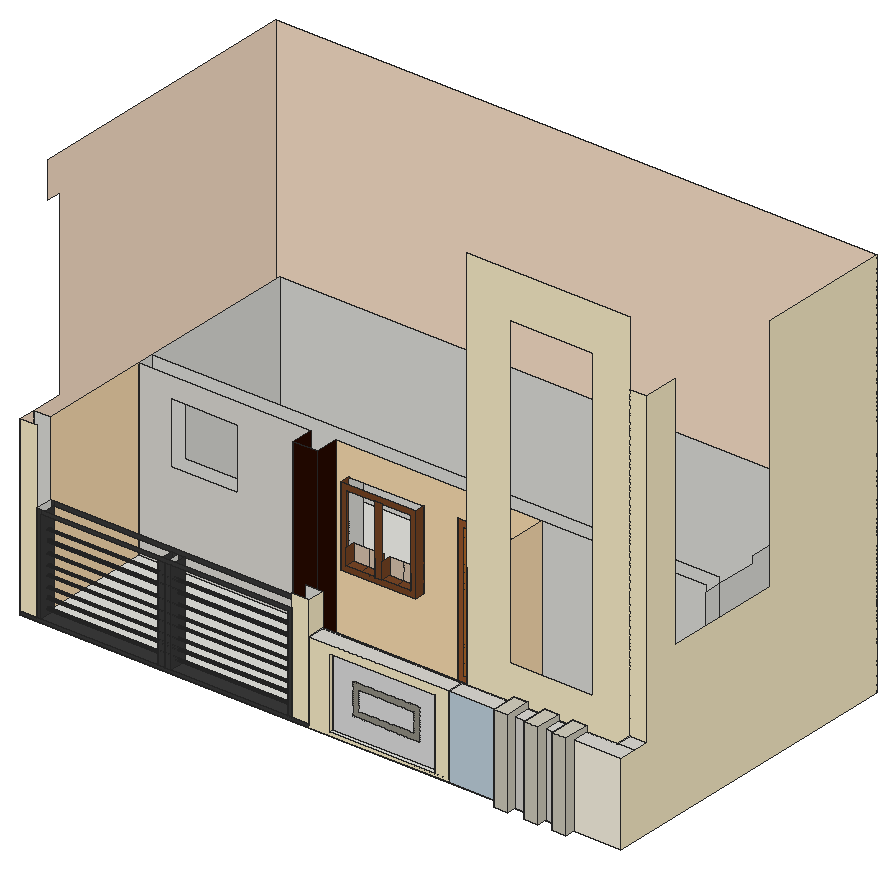
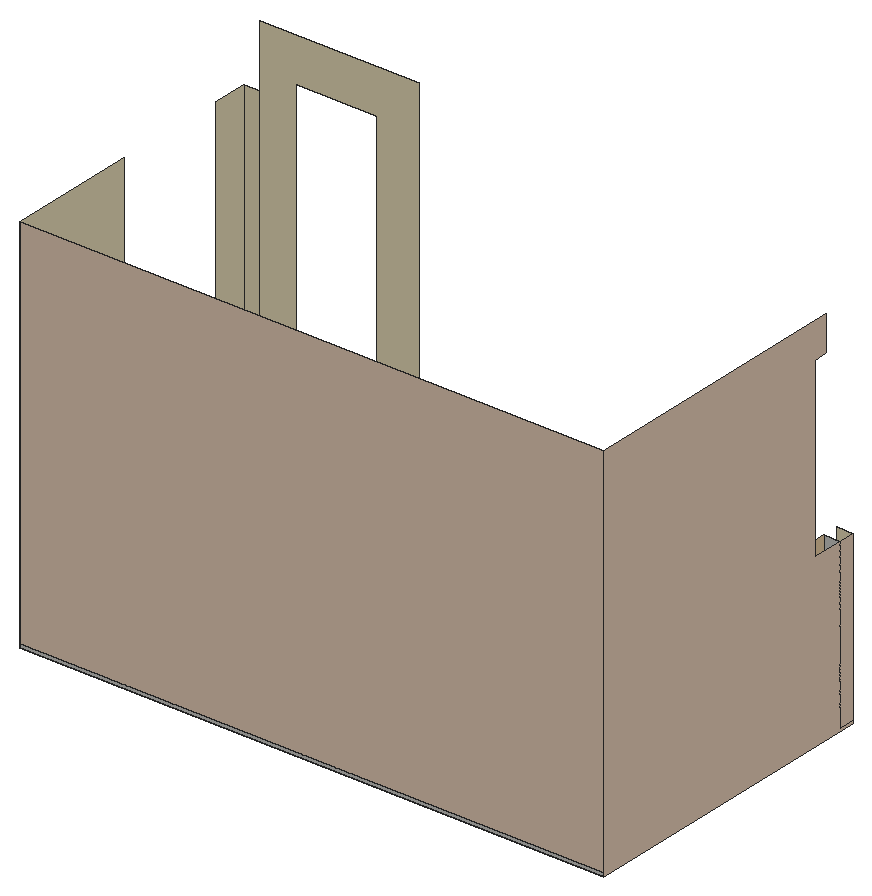
# SketchUp Ruby script. Lengths in inches.
U = 1.inch
M = Sketchup.active_model
def pt(a) = Geom::Point3d.new(a.map { |v| v * U })
def face(e, loops, mat)
  f = e.add_face(loops[0].map { |a| pt(a) })
  loops[1..].each { |l| e.add_face(l.map { |a| pt(a) }).erase! }
  f.material = f.back_material = mat if mat
  f
end
# faces: each face lists its corners as indices into pts; further lists are holes
def faces(e, pts, list, mat = nil) = list.each { |f| face(e, (f[0].is_a?(Array) ? f : [f]).map { |l| l.map { |i| pts[i] } }, mat) }
# xy, xz, yz: faces in a plane at the given z, y or x. An outline is a flat list of corners, or four numbers for a rectangle; further outlines are holes
def ring(l) = l.size == 4 ? [[l[0], l[1]], [l[2], l[1]], [l[2], l[3]], [l[0], l[3]]] : l.each_slice(2).to_a
def flat(e, list, mat, &to3) = list.each { |f| face(e, (f[0].is_a?(Array) ? f : [f]).map { |l| ring(l).map { |u, v| to3.(u, v) } }, mat) }
def xy(e, z, list, mat = nil) = flat(e, list, mat) { |x, y| [x, y, z] }
def xz(e, y, list, mat = nil) = flat(e, list, mat) { |x, z| [x, y, z] }
def yz(e, x, list, mat = nil) = flat(e, list, mat) { |y, z| [x, y, z] }
def lines(e, pts, list) = list.each { |a, b| e.add_line(pt(pts[a]), pt(pts[b])) }
# prism: a flat outline (further loops are holes) pulled along v
def prism(e, loops, v, mat = nil)
  f = face(e, loops, mat); d = Geom::Vector3d.new(v.map { |x| x * U })
  f.pushpull(f.normal.samedirection?(d) ? d.length : -d.length)
end
def box(e, o, s, mat = nil) = prism(e, [[o, [o[0] + s[0], o[1], o[2]], [o[0] + s[0], o[1] + s[1], o[2]], [o[0], o[1] + s[1], o[2]]]], [0, 0, s[2]], mat)
def at(x, y, z, deg = 0) = Geom::Transformation.translation(pt([x, y, z])) * Geom::Transformation.rotation(ORIGIN, Z_AXIS, deg.degrees)
def axes(o, x, y, z) = Geom::Transformation.new([*x, 0, *y, 0, *z, 0, *pt(o).to_a, 1])
def part(name) = M.definitions.add(name)
# library, detail: a bought-in or finely detailed component or shape, given as its bounding box
def library(name, o, s) = part(name).tap { |d| box(d.entities, o, s) }
def detail(e, o, s) = box(e.add_group.entities, o, s)
def put(e, d, t, mat = nil) = e.add_instance(d, t).tap { |i| i.material = mat if mat }
def group(e, t, mat = nil) = e.add_group.tap { |g| g.transformation = t; g.material = mat if mat }.entities
root = M.entities
M.materials.add("[Color B08]").color = [40, 10, 0]
M.materials.add("[Color C01]").color = [221, 199, 177]
M.materials.add("[Color C01]1").color = [255, 229, 204]
M.materials.add("[Color D01]").color = [255, 242, 204]
M.materials.add("[Color M01]").color = [226, 226, 226]
M.materials.add("[Color M07]").color = [58, 58, 58]
M.materials.add("[Formica Beige]").color = [255, 225, 180]
M.materials.add("[Formica Graystone]").color = [211, 207, 191]
M.materials.add("[Formica Graystone]1").color = [255, 249, 231]
M.materials.add("[Formica Graystone]2").color = [149, 146, 135]
M.materials.add("[Formica Laminate Dark]").color = [50, 53, 60]
M.materials.add("[Marble Carrara Gold Floor Tile]").color = [225, 223, 217]
M.materials.add("[Terrazzo Light Blue]").color = [196, 214, 227]
M.materials.add("[Terrazzo Tile Light]").color = [219, 217, 210]
M.materials.add("[Wood Bamboo]").color = [177, 105, 43]
M.materials.add("[Wood Cherry Original]").color = [152, 86, 42]
M.materials.add("[Wood Floor Light]").color = [204, 176, 127]
M.materials.add("[Wood Veneer 01]").color = [120, 70, 37]
xy(root,0,[[1538.08,0,1538.08,25.9375,0,25.9375,0,938.08,1713.03,938.08,1713.03,25.9375,1578.55,25.9375,1578.55,0],[1370.58,0,1411.05,25.9375],[1458.08,0,1498.55,25.9375]])
xy(root,9,[[0,25.9375,0,73.63,1665.33,73.63,1665.33,119.17,1198.27,119.17,1198.27,388.54,609.42,388.54,609.42,324.79,539.84,324.79,539.84,388.54,47.7,388.54,47.7,25.9375],[47.7,25.9375,58.17,73.63],[392.86,25.9375,411.53,73.63],[411.53,25.9375,430.19,73.63],[763.2,25.9375,775.53,73.63],
  [775.53,25.9375,824.4,73.63],[882.08,25.9375,1183.86,38.5625],[1183.86,25.9375,1222.55,73.63],[882.08,38.5625,1183.86,73.63],[958.75,388.54,1164.68,436.38],
  [47.7,436.38,1665.33,890.39]])
xy(root,9,[[58.17,25.9375,392.86,73.63],[430.19,25.9375,763.2,73.63]],"[Color M07]")
xy(root,195.52,[[648.52,388.54,860.65,436.38]])
xy(root,195.52,[[648.52,359.29,860.65,388.54]],"[Wood Veneer 01]")
xy(root,209.32,[[882.08,25.9375,1183.86,38.5625]],"[Color D01]")
xy(root,209.8125,[[662.82,359.29,704.31,388.54],[704.31,359.29,745.81,388.54],[764.54,359.29,805.45,388.54],[805.45,359.29,846.36,388.54]],"[Wood Veneer 01]")
xy(root,233.1875,[[1370.58,25.9375,1411.05,73.63],[1458.08,25.9375,1498.55,73.63]])
xy(root,233.1875,[[824.4,25.9375,1222.55,73.63],[1222.55,25.9375,1370.58,73.63],[1411.05,25.9375,1458.08,73.63],[1498.55,25.9375,1538.08,73.63],[1578.55,25.9375,1713.03,73.63],
  [1665.33,73.63,1713.03,119.17]],"[Terrazzo Tile Light]")
xy(root,249.75,[[1370.58,0,1411.05,73.63],[1458.08,0,1498.55,73.63],[1538.08,0,1578.55,73.63]],"[Formica Graystone]")
xz(root,0,[[1370.58,0,1411.05,249.75],[1458.08,0,1498.55,249.75],[1538.08,0,1578.55,249.75]],"[Formica Graystone]")
xz(root,25.9375,[[1370.58,0,1411.05,233.1875],[1458.08,0,1498.55,233.1875]])
xz(root,25.9375,[[824.4,0,1222.55,0,1222.55,9,882.08,9,882.08,209.32,1183.86,209.32,1183.86,9,1222.55,9,1222.55,233.1875,824.4,233.1875],[0,9,47.7,500.125],[775.53,9,824.4,326.25]],"[Color D01]")
xz(root,25.9375,[[0,0,824.4,9],[47.7,9,58.17,288.4375],[763.2,9,775.53,9,775.53,288.4375,58.17,288.4375,58.17,276.5625,763.2,276.5625],[392.86,9,411.53,276.5625],[411.53,9,430.19,276.5625]],"[Color M07]")
xz(root,25.9375,[[1578.55,0,1713.03,233.1875]],"[Formica Graystone]1")
xz(root,25.9375,[[1222.55,0,1370.58,233.1875]],"[Terrazzo Light Blue]")
xz(root,25.9375,[[1411.05,0,1458.08,233.1875],[1498.55,0,1538.08,233.1875]],"[Terrazzo Tile Light]")
xz(root,38.5625,[[[882.08,9,1183.86,209.32],[939.22,64.12,1130.16,154.99]],[957.24,82.13,1112.14,136.97]],"[Color M01]")
xz(root,38.5625,[[[939.22,64.12,1130.16,154.99],[957.24,82.13,1112.14,136.97]]],"[Formica Graystone]2")
xz(root,73.63,[[0,9,47.7,500.125],[775.53,9,824.4,326.25],[824.4,9,882.08,233.1875],[1183.86,9,1183.86,209.32,882.08,209.32,882.08,233.1875,1222.55,233.1875,1222.55,9],[882.08,9,1183.86,209.32]])
xz(root,73.63,[[47.7,9,58.17,288.4375],[763.2,9,763.2,276.5625,58.17,276.5625,58.17,288.4375,775.53,288.4375,775.53,9],[392.86,9,411.53,276.5625],[411.53,9,430.19,276.5625]],"[Color M07]")
xz(root,73.63,[[1222.55,9,1222.55,233.1875,1538.08,233.1875,1538.08,249.75,1578.55,249.75,1578.55,233.1875,1665.33,233.1875,1665.33,9],[1370.58,233.1875,1411.05,249.75],[1458.08,233.1875,1498.55,249.75]],"[Formica Graystone]")
xz(root,119.17,[[[1198.27,9,1665.33,1305.375],[1322.15,298.625,1559.21,1175.6875]],[1665.33,233.1875,1713.03,1119.0625]],"[Color D01]")
xz(root,324.79,[[539.84,9,609.42,500.125]],"[Color B08]")
xz(root,359.29,[[[648.52,195.52,860.65,420.08],[662.82,209.8125,846.36,405.79]],[745.81,209.8125,764.54,405.79]],"[Wood Veneer 01]")
xz(root,388.54,[[1198.27,9,1665.33,500.125]])
xz(root,388.54,[[662.82,209.8125,704.31,256.87],[704.31,209.8125,745.81,256.87],[764.54,209.8125,805.45,256.87],[805.45,209.8125,846.36,256.87]],"[Color C01]")
xz(root,388.54,[[[609.42,9,958.75,9,958.75,423.9375,1164.68,423.9375,1164.68,9,1198.27,9,1198.27,500.125,609.42,500.125],[648.52,195.52,860.65,420.08]]],"[Formica Beige]")
xz(root,388.54,[[[47.7,9,539.84,500.125],[139.94,267,331.76,443.06]]],"[Marble Carrara Gold Floor Tile]")
xz(root,388.54,[[[976.52,26.77,1146.91,406.17],[984.3,166.91,996.99,249.85]]],"[Wood Bamboo]")
xz(root,388.54,[[[958.75,9,1164.68,423.9375],[976.52,26.77,1146.91,406.17]]],"[Wood Cherry Original]")
xz(root,388.54,[[984.3,166.91,996.99,249.85]],"[Wood Floor Light]")
xz(root,436.38,[[[47.7,9,47.7,500.125,1665.33,500.125,1665.33,9,1164.68,9,1164.68,423.9375,958.75,423.9375,958.75,9],[648.52,195.52,860.65,420.08],[139.94,267,331.76,443.06]]])
xz(root,890.39,[[47.7,9,1665.33,500.125]])
xz(root,938.08,[[0,0,1713.03,9]])
xz(root,938.08,[[0,9,1713.03,1119.0625]],"[Color C01]1")
yz(root,0,[[25.9375,0,25.9375,9,73.63,9,73.63,500.125,166.1,500.125,166.1,1016.9375,122.54,1016.9375,122.54,1119.0625,938.08,1119.0625,938.08,0],[25.9375,9,73.63,500.125]],"[Color C01]1")
yz(root,47.7,[[25.9375,9,73.63,288.4375],[388.54,9,436.38,500.125],[436.38,9,890.39,500.125]])
yz(root,47.7,[[73.63,9,388.54,500.125]],"[Formica Beige]")
yz(root,58.17,[[51.27,21.94,50.49,22.04,49.77,22.34,49.15,22.82,48.67,23.44,48.37,24.16,48.27,24.94,48.37,25.72,48.67,26.44,49.15,27.0625,49.77,27.54,50.49,27.84,51.27,27.94,52.04,27.84,52.77,27.54,53.39,27.0625,53.87,26.44,54.17,25.72,54.27,24.94,54.17,24.16,53.87,23.44,53.39,22.82,52.77,22.34,52.04,22.04],[51.27,49.25,50.49,49.35,49.77,49.65,49.15,50.13,48.67,50.75,48.37,51.48,48.27,52.25,48.37,53.03,48.67,53.75,49.15,54.375,49.77,54.85,50.49,55.15,51.27,55.25,52.04,55.15,52.77,54.85,53.39,54.375,53.87,53.75,54.17,53.03,54.27,52.25,54.17,51.48,53.87,50.75,53.39,50.13,52.77,49.65,52.04,49.35],[51.27,76.69,50.49,76.79,49.77,77.09,49.15,77.57,48.67,78.19,48.37,78.91,48.27,79.69,48.37,80.47,48.67,81.19,49.15,81.8125,49.77,82.29,50.49,82.59,51.27,82.69,52.04,82.59,52.77,82.29,53.39,81.8125,53.87,81.19,54.17,80.47,54.27,79.69,54.17,78.91,53.87,78.19,53.39,77.57,52.77,77.09,52.04,76.79],[51.27,107.44,50.49,107.54,49.77,107.84,49.15,108.32,48.67,108.94,48.37,109.66,48.27,110.44,48.37,111.22,48.67,111.94,49.15,112.5625,49.77,113.04,50.49,113.34,51.27,113.44,52.04,113.34,52.77,113.04,53.39,112.5625,53.87,111.94,54.17,111.22,54.27,110.44,54.17,109.66,53.87,108.94,53.39,108.32,52.77,107.84,52.04,107.54],[51.27,132.75,50.49,132.85,49.77,133.15,49.15,133.63,48.67,134.25,48.37,134.98,48.27,135.75,48.37,136.53,48.67,137.25,49.15,137.875,49.77,138.35,50.49,138.65,51.27,138.75,52.04,138.65,52.77,138.35,53.39,137.875,53.87,137.25,54.17,136.53,54.27,135.75,54.17,134.98,53.87,134.25,53.39,133.63,52.77,133.15,52.04,132.85],
  [51.27,163.5,50.49,163.6,49.77,163.9,49.15,164.38,48.67,165,48.37,165.73,48.27,166.5,48.37,167.28,48.67,168,49.15,168.625,49.77,169.1,50.49,169.4,51.27,169.5,52.04,169.4,52.77,169.1,53.39,168.625,53.87,168,54.17,167.28,54.27,166.5,54.17,165.73,53.87,165,53.39,164.38,52.77,163.9,52.04,163.6],[51.27,195.56,50.49,195.67,49.77,195.97,49.15,196.44,48.67,197.06,48.37,197.79,48.27,198.56,48.37,199.34,48.67,200.06,49.15,200.6875,49.77,201.16,50.49,201.46,51.27,201.56,52.04,201.46,52.77,201.16,53.39,200.6875,53.87,200.06,54.17,199.34,54.27,198.56,54.17,197.79,53.87,197.06,53.39,196.44,52.77,195.97,52.04,195.67],[51.27,225.44,50.49,225.54,49.77,225.84,49.15,226.32,48.67,226.94,48.37,227.66,48.27,228.44,48.37,229.22,48.67,229.94,49.15,230.5625,49.77,231.04,50.49,231.34,51.27,231.44,52.04,231.34,52.77,231.04,53.39,230.5625,53.87,229.94,54.17,229.22,54.27,228.44,54.17,227.66,53.87,226.94,53.39,226.32,52.77,225.84,52.04,225.54]])
yz(root,58.17,[[[25.9375,9,73.63,276.5625],[51.27,21.94,50.49,22.04,49.77,22.34,49.15,22.82,48.67,23.44,48.37,24.16,48.27,24.94,48.37,25.72,48.67,26.44,49.15,27.0625,49.77,27.54,50.49,27.84,51.27,27.94,52.04,27.84,52.77,27.54,53.39,27.0625,53.87,26.44,54.17,25.72,54.27,24.94,54.17,24.16,53.87,23.44,53.39,22.82,52.77,22.34,52.04,22.04],[51.27,225.44,50.49,225.54,49.77,225.84,49.15,226.32,48.67,226.94,48.37,227.66,48.27,228.44,48.37,229.22,48.67,229.94,49.15,230.5625,49.77,231.04,50.49,231.34,51.27,231.44,52.04,231.34,52.77,231.04,53.39,230.5625,53.87,229.94,54.17,229.22,54.27,228.44,54.17,227.66,53.87,226.94,53.39,226.32,52.77,225.84,52.04,225.54],[51.27,49.25,50.49,49.35,49.77,49.65,49.15,50.13,48.67,50.75,48.37,51.48,48.27,52.25,48.37,53.03,48.67,53.75,49.15,54.375,49.77,54.85,50.49,55.15,51.27,55.25,52.04,55.15,52.77,54.85,53.39,54.375,53.87,53.75,54.17,53.03,54.27,52.25,54.17,51.48,53.87,50.75,53.39,50.13,52.77,49.65,52.04,49.35],[51.27,195.56,50.49,195.67,49.77,195.97,49.15,196.44,48.67,197.06,48.37,197.79,48.27,198.56,48.37,199.34,48.67,200.06,49.15,200.6875,49.77,201.16,50.49,201.46,51.27,201.56,52.04,201.46,52.77,201.16,53.39,200.6875,53.87,200.06,54.17,199.34,54.27,198.56,54.17,197.79,53.87,197.06,53.39,196.44,52.77,195.97,52.04,195.67],[51.27,107.44,50.49,107.54,49.77,107.84,49.15,108.32,48.67,108.94,48.37,109.66,48.27,110.44,48.37,111.22,48.67,111.94,49.15,112.5625,49.77,113.04,50.49,113.34,51.27,113.44,52.04,113.34,52.77,113.04,53.39,112.5625,53.87,111.94,54.17,111.22,54.27,110.44,54.17,109.66,53.87,108.94,53.39,108.32,52.77,107.84,52.04,107.54],[51.27,163.5,50.49,163.6,49.77,163.9,49.15,164.38,48.67,165,48.37,165.73,48.27,166.5,48.37,167.28,48.67,168,49.15,168.625,49.77,169.1,50.49,169.4,51.27,169.5,52.04,169.4,52.77,169.1,53.39,168.625,53.87,168,54.17,167.28,54.27,166.5,54.17,165.73,53.87,165,53.39,164.38,52.77,163.9,52.04,163.6],[51.27,132.75,50.49,132.85,49.77,133.15,49.15,133.63,48.67,134.25,48.37,134.98,48.27,135.75,48.37,136.53,48.67,137.25,49.15,137.875,49.77,138.35,50.49,138.65,51.27,138.75,52.04,138.65,52.77,138.35,53.39,137.875,53.87,137.25,54.17,136.53,54.27,135.75,54.17,134.98,53.87,134.25,53.39,133.63,52.77,133.15,52.04,132.85],[51.27,76.69,50.49,76.79,49.77,77.09,49.15,77.57,48.67,78.19,48.37,78.91,48.27,79.69,48.37,80.47,48.67,81.19,49.15,81.8125,49.77,82.29,50.49,82.59,51.27,82.69,52.04,82.59,52.77,82.29,53.39,81.8125,53.87,81.19,54.17,80.47,54.27,79.69,54.17,78.91,53.87,78.19,53.39,77.57,52.77,77.09,52.04,76.79],[51.27,251.25,50.49,251.35,49.77,251.65,49.15,252.13,48.67,252.75,48.37,253.48,48.27,254.25,48.37,255.03,48.67,255.75,49.15,256.375,49.77,256.85,50.49,257.15,51.27,257.25,52.04,257.15,52.77,256.85,53.39,256.375,53.87,255.75,54.17,255.03,54.27,254.25,54.17,253.48,53.87,252.75,53.39,252.13,52.77,251.65,52.04,251.35]]],"[Color M07]")
yz(root,392.86,[[25.9375,9,73.63,276.5625]],"[Color M07]")
yz(root,411.53,[[25.9375,9,73.63,276.5625]])
yz(root,430.19,[[25.9375,9,73.63,276.5625]],"[Color M07]")
yz(root,539.84,[[324.79,9,388.54,500.125]],"[Color B08]")
yz(root,609.42,[[324.79,9,388.54,500.125]],"[Color B08]")
yz(root,648.52,[[388.54,195.52,436.38,420.08]])
yz(root,648.52,[[359.29,195.52,388.54,420.08]],"[Wood Veneer 01]")
yz(root,662.82,[[359.29,209.8125,388.54,256.87]],"[Wood Veneer 01]")
yz(root,745.81,[[359.29,209.8125,388.54,256.87]],"[Wood Veneer 01]")
yz(root,763.2,[[[25.9375,9,73.63,276.5625],[51.27,251.25,52.04,251.35,52.77,251.65,53.39,252.13,53.87,252.75,54.17,253.48,54.27,254.25,54.17,255.03,53.87,255.75,53.39,256.375,52.77,256.85,52.04,257.15,51.27,257.25,50.49,257.15,49.77,256.85,49.15,256.375,48.67,255.75,48.37,255.03,48.27,254.25,48.37,253.48,48.67,252.75,49.15,252.13,49.77,251.65,50.49,251.35],[51.27,225.44,52.04,225.54,52.77,225.84,53.39,226.32,53.87,226.94,54.17,227.66,54.27,228.44,54.17,229.22,53.87,229.94,53.39,230.5625,52.77,231.04,52.04,231.34,51.27,231.44,50.49,231.34,49.77,231.04,49.15,230.5625,48.67,229.94,48.37,229.22,48.27,228.44,48.37,227.66,48.67,226.94,49.15,226.32,49.77,225.84,50.49,225.54],[51.27,195.56,52.04,195.67,52.77,195.97,53.39,196.44,53.87,197.06,54.17,197.79,54.27,198.56,54.17,199.34,53.87,200.06,53.39,200.6875,52.77,201.16,52.04,201.46,51.27,201.56,50.49,201.46,49.77,201.16,49.15,200.6875,48.67,200.06,48.37,199.34,48.27,198.56,48.37,197.79,48.67,197.06,49.15,196.44,49.77,195.97,50.49,195.67],[51.27,163.5,52.04,163.6,52.77,163.9,53.39,164.38,53.87,165,54.17,165.73,54.27,166.5,54.17,167.28,53.87,168,53.39,168.625,52.77,169.1,52.04,169.4,51.27,169.5,50.49,169.4,49.77,169.1,49.15,168.625,48.67,168,48.37,167.28,48.27,166.5,48.37,165.73,48.67,165,49.15,164.38,49.77,163.9,50.49,163.6],[51.27,132.75,52.04,132.85,52.77,133.15,53.39,133.63,53.87,134.25,54.17,134.98,54.27,135.75,54.17,136.53,53.87,137.25,53.39,137.875,52.77,138.35,52.04,138.65,51.27,138.75,50.49,138.65,49.77,138.35,49.15,137.875,48.67,137.25,48.37,136.53,48.27,135.75,48.37,134.98,48.67,134.25,49.15,133.63,49.77,133.15,50.49,132.85],[51.27,107.44,52.04,107.54,52.77,107.84,53.39,108.32,53.87,108.94,54.17,109.66,54.27,110.44,54.17,111.22,53.87,111.94,53.39,112.5625,52.77,113.04,52.04,113.34,51.27,113.44,50.49,113.34,49.77,113.04,49.15,112.5625,48.67,111.94,48.37,111.22,48.27,110.44,48.37,109.66,48.67,108.94,49.15,108.32,49.77,107.84,50.49,107.54],[51.27,76.69,52.04,76.79,52.77,77.09,53.39,77.57,53.87,78.19,54.17,78.91,54.27,79.69,54.17,80.47,53.87,81.19,53.39,81.8125,52.77,82.29,52.04,82.59,51.27,82.69,50.49,82.59,49.77,82.29,49.15,81.8125,48.67,81.19,48.37,80.47,48.27,79.69,48.37,78.91,48.67,78.19,49.15,77.57,49.77,77.09,50.49,76.79],[51.27,49.25,52.04,49.35,52.77,49.65,53.39,50.13,53.87,50.75,54.17,51.48,54.27,52.25,54.17,53.03,53.87,53.75,53.39,54.375,52.77,54.85,52.04,55.15,51.27,55.25,50.49,55.15,49.77,54.85,49.15,54.375,48.67,53.75,48.37,53.03,48.27,52.25,48.37,51.48,48.67,50.75,49.15,50.13,49.77,49.65,50.49,49.35],[51.27,21.94,52.04,22.04,52.77,22.34,53.39,22.82,53.87,23.44,54.17,24.16,54.27,24.94,54.17,25.72,53.87,26.44,53.39,27.0625,52.77,27.54,52.04,27.84,51.27,27.94,50.49,27.84,49.77,27.54,49.15,27.0625,48.67,26.44,48.37,25.72,48.27,24.94,48.37,24.16,48.67,23.44,49.15,22.82,49.77,22.34,50.49,22.04]]],"[Color M07]")
yz(root,764.54,[[359.29,209.8125,388.54,256.87]],"[Wood Veneer 01]")
yz(root,775.53,[[25.9375,9,73.63,288.4375]])
yz(root,824.4,[[25.9375,9,73.63,233.1875]])
yz(root,824.4,[[25.9375,233.1875,73.63,326.25]],"[Color D01]")
yz(root,846.36,[[359.29,209.8125,388.54,256.87]],"[Wood Veneer 01]")
yz(root,860.65,[[388.54,195.52,436.38,420.08]])
yz(root,860.65,[[359.29,195.52,388.54,420.08]],"[Wood Veneer 01]")
yz(root,882.08,[[38.5625,9,73.63,209.32]])
yz(root,882.08,[[25.9375,9,38.5625,209.32]],"[Color D01]")
yz(root,958.75,[[388.54,9,436.38,423.9375]])
yz(root,1164.68,[[388.54,9,436.38,423.9375]])
yz(root,1183.86,[[38.5625,9,73.63,209.32]])
yz(root,1183.86,[[25.9375,9,38.5625,209.32]],"[Color D01]")
yz(root,1198.27,[[119.17,9,388.54,500.125]],"[Formica Beige]")
yz(root,1222.55,[[25.9375,9,73.63,233.1875]])
yz(root,1370.58,[[0,0,0,249.75,73.63,249.75,73.63,233.1875,25.9375,233.1875,25.9375,0]],"[Formica Graystone]")
yz(root,1411.05,[[0,0,25.9375,0,25.9375,233.1875,73.63,233.1875,73.63,249.75,0,249.75]],"[Formica Graystone]")
yz(root,1458.08,[[0,0,0,249.75,73.63,249.75,73.63,233.1875,25.9375,233.1875,25.9375,0]],"[Formica Graystone]")
yz(root,1498.55,[[0,0,25.9375,0,25.9375,233.1875,73.63,233.1875,73.63,249.75,0,249.75]],"[Formica Graystone]")
yz(root,1538.08,[[0,0,0,249.75,73.63,249.75,73.63,233.1875,25.9375,233.1875,25.9375,0]],"[Formica Graystone]")
yz(root,1578.55,[[0,0,25.9375,0,25.9375,233.1875,73.63,233.1875,73.63,249.75,0,249.75]],"[Formica Graystone]")
yz(root,1665.33,[[73.63,9,119.17,233.1875],[388.54,9,436.38,481.82],[436.38,9,436.38,481.82,557.62,481.82,557.62,500.125,890.39,500.125,890.39,9]])
yz(root,1713.03,[[25.9375,0,938.08,0,938.08,1119.0625,557.62,1119.0625,557.62,438.77,219.81,438.77,219.81,1119.0625,119.17,1119.0625,119.17,233.1875,25.9375,233.1875]],"[Color D01]")
p = [[58.17,50.49,22.04],[58.17,51.27,21.94],[763.2,51.27,21.94],[763.2,50.49,22.04],[58.17,52.04,22.04],[763.2,52.04,22.04],
  [58.17,49.77,22.34],[763.2,49.77,22.34],[58.17,52.77,22.34],[763.2,52.77,22.34],[58.17,49.15,22.82],[763.2,49.15,22.82],
  [58.17,53.39,22.82],[763.2,53.39,22.82],[58.17,48.67,23.44],[763.2,48.67,23.44],[58.17,53.87,23.44],[763.2,53.87,23.44],
  [58.17,48.37,24.16],[763.2,48.37,24.16],[58.17,54.17,24.16],[763.2,54.17,24.16],[58.17,48.27,24.94],[763.2,48.27,24.94],
  [58.17,54.27,24.94],[763.2,54.27,24.94],[58.17,48.37,25.72],[763.2,48.37,25.72],[58.17,54.17,25.72],[763.2,54.17,25.72],
  [58.17,48.67,26.44],[763.2,48.67,26.44],[58.17,53.87,26.44],[763.2,53.87,26.44],[58.17,49.15,27.0625],[763.2,49.15,27.0625],
  [58.17,53.39,27.0625],[763.2,53.39,27.0625],[58.17,49.77,27.54],[763.2,49.77,27.54],[58.17,52.77,27.54],[763.2,52.77,27.54],
  [58.17,50.49,27.84],[763.2,50.49,27.84],[58.17,52.04,27.84],[763.2,52.04,27.84],[58.17,51.27,27.94],[763.2,51.27,27.94],
  [58.17,50.49,49.35],[58.17,51.27,49.25],[763.2,51.27,49.25],[763.2,50.49,49.35],[58.17,52.04,49.35],[763.2,52.04,49.35],
  [58.17,49.77,49.65],[763.2,49.77,49.65],[58.17,52.77,49.65],[763.2,52.77,49.65],[58.17,49.15,50.13],[763.2,49.15,50.13],
  [58.17,53.39,50.13],[763.2,53.39,50.13],[58.17,48.67,50.75],[763.2,48.67,50.75],[58.17,53.87,50.75],[763.2,53.87,50.75],
  [58.17,48.37,51.48],[763.2,48.37,51.48],[58.17,54.17,51.48],[763.2,54.17,51.48],[58.17,48.27,52.25],[763.2,48.27,52.25],
  [58.17,54.27,52.25],[763.2,54.27,52.25],[58.17,48.37,53.03],[763.2,48.37,53.03],[58.17,54.17,53.03],[763.2,54.17,53.03],
  [58.17,48.67,53.75],[763.2,48.67,53.75],[58.17,53.87,53.75],[763.2,53.87,53.75],[58.17,49.15,54.375],[763.2,49.15,54.375],
  [58.17,53.39,54.375],[763.2,53.39,54.375],[58.17,49.77,54.85],[763.2,49.77,54.85],[58.17,52.77,54.85],[763.2,52.77,54.85],
  [58.17,50.49,55.15],[763.2,50.49,55.15],[58.17,52.04,55.15],[763.2,52.04,55.15],[58.17,51.27,55.25],[763.2,51.27,55.25],
  [58.17,50.49,76.79],[58.17,51.27,76.69],[763.2,51.27,76.69],[763.2,50.49,76.79],[58.17,52.04,76.79],[763.2,52.04,76.79],
  [58.17,49.77,77.09],[763.2,49.77,77.09],[58.17,52.77,77.09],[763.2,52.77,77.09],[58.17,49.15,77.57],[763.2,49.15,77.57],
  [58.17,53.39,77.57],[763.2,53.39,77.57],[58.17,48.67,78.19],[763.2,48.67,78.19],[58.17,53.87,78.19],[763.2,53.87,78.19],
  [58.17,48.37,78.91],[763.2,48.37,78.91],[58.17,54.17,78.91],[763.2,54.17,78.91],[58.17,48.27,79.69],[763.2,48.27,79.69],
  [58.17,54.27,79.69],[763.2,54.27,79.69],[58.17,48.37,80.47],[763.2,48.37,80.47],[58.17,54.17,80.47],[763.2,54.17,80.47],
  [58.17,48.67,81.19],[763.2,48.67,81.19],[58.17,53.87,81.19],[763.2,53.87,81.19],[58.17,49.15,81.8125],[763.2,49.15,81.8125],
  [58.17,53.39,81.8125],[763.2,53.39,81.8125],[58.17,49.77,82.29],[763.2,49.77,82.29],[58.17,52.77,82.29],[763.2,52.77,82.29],
  [58.17,50.49,82.59],[763.2,50.49,82.59],[58.17,52.04,82.59],[763.2,52.04,82.59],[58.17,51.27,82.69],[763.2,51.27,82.69],
  [58.17,50.49,107.54],[58.17,51.27,107.44],[763.2,51.27,107.44],[763.2,50.49,107.54],[58.17,52.04,107.54],[763.2,52.04,107.54],
  [58.17,49.77,107.84],[763.2,49.77,107.84],[58.17,52.77,107.84],[763.2,52.77,107.84],[58.17,49.15,108.32],[763.2,49.15,108.32],
  [58.17,53.39,108.32],[763.2,53.39,108.32],[58.17,48.67,108.94],[763.2,48.67,108.94],[58.17,53.87,108.94],[763.2,53.87,108.94],
  [58.17,48.37,109.66],[763.2,48.37,109.66],[58.17,54.17,109.66],[763.2,54.17,109.66],[58.17,48.27,110.44],[763.2,48.27,110.44],
  [58.17,54.27,110.44],[763.2,54.27,110.44],[58.17,48.37,111.22],[763.2,48.37,111.22],[58.17,54.17,111.22],[763.2,54.17,111.22],
  [58.17,48.67,111.94],[763.2,48.67,111.94],[58.17,53.87,111.94],[763.2,53.87,111.94],[58.17,49.15,112.5625],[763.2,49.15,112.5625],
  [58.17,53.39,112.5625],[763.2,53.39,112.5625],[58.17,49.77,113.04],[763.2,49.77,113.04],[58.17,52.77,113.04],[763.2,52.77,113.04],
  [58.17,50.49,113.34],[763.2,50.49,113.34],[58.17,52.04,113.34],[763.2,52.04,113.34],[58.17,51.27,113.44],[763.2,51.27,113.44],
  [58.17,50.49,132.85],[58.17,51.27,132.75],[763.2,51.27,132.75],[763.2,50.49,132.85],[58.17,52.04,132.85],[763.2,52.04,132.85],
  [58.17,49.77,133.15],[763.2,49.77,133.15],[58.17,52.77,133.15],[763.2,52.77,133.15],[58.17,49.15,133.63],[763.2,49.15,133.63],
  [58.17,53.39,133.63],[763.2,53.39,133.63],[58.17,48.67,134.25],[763.2,48.67,134.25],[58.17,53.87,134.25],[763.2,53.87,134.25],
  [58.17,48.37,134.98],[763.2,48.37,134.98],[58.17,54.17,134.98],[763.2,54.17,134.98],[58.17,48.27,135.75],[763.2,48.27,135.75],
  [58.17,54.27,135.75],[763.2,54.27,135.75],[58.17,48.37,136.53],[763.2,48.37,136.53],[58.17,54.17,136.53],[763.2,54.17,136.53],
  [58.17,48.67,137.25],[763.2,48.67,137.25],[58.17,53.87,137.25],[763.2,53.87,137.25],[58.17,49.15,137.875],[763.2,49.15,137.875],
  [58.17,53.39,137.875],[763.2,53.39,137.875],[58.17,49.77,138.35],[763.2,49.77,138.35],[58.17,52.77,138.35],[763.2,52.77,138.35],
  [58.17,50.49,138.65],[763.2,50.49,138.65],[58.17,52.04,138.65],[763.2,52.04,138.65],[58.17,51.27,138.75],[763.2,51.27,138.75],
  [58.17,50.49,163.6],[58.17,51.27,163.5],[763.2,51.27,163.5],[763.2,50.49,163.6],[58.17,52.04,163.6],[763.2,52.04,163.6],
  [58.17,49.77,163.9],[763.2,49.77,163.9],[58.17,52.77,163.9],[763.2,52.77,163.9],[58.17,49.15,164.38],[763.2,49.15,164.38],
  [58.17,53.39,164.38],[763.2,53.39,164.38],[58.17,48.67,165],[763.2,48.67,165],[58.17,53.87,165],[763.2,53.87,165],
  [58.17,48.37,165.73],[763.2,48.37,165.73],[58.17,54.17,165.73],[763.2,54.17,165.73],[58.17,48.27,166.5],[763.2,48.27,166.5],
  [58.17,54.27,166.5],[763.2,54.27,166.5],[58.17,48.37,167.28],[763.2,48.37,167.28],[58.17,54.17,167.28],[763.2,54.17,167.28],
  [58.17,48.67,168],[763.2,48.67,168],[58.17,53.87,168],[763.2,53.87,168],[58.17,49.15,168.625],[763.2,49.15,168.625],
  [58.17,53.39,168.625],[763.2,53.39,168.625],[58.17,49.77,169.1],[763.2,49.77,169.1],[58.17,52.77,169.1],[763.2,52.77,169.1],
  [58.17,50.49,169.4],[763.2,50.49,169.4],[58.17,52.04,169.4],[763.2,52.04,169.4],[58.17,51.27,169.5],[763.2,51.27,169.5],
  [58.17,50.49,195.67],[58.17,51.27,195.56],[763.2,51.27,195.56],[763.2,50.49,195.67],[58.17,52.04,195.67],[763.2,52.04,195.67],
  [58.17,49.77,195.97],[763.2,49.77,195.97],[58.17,52.77,195.97],[763.2,52.77,195.97],[58.17,49.15,196.44],[763.2,49.15,196.44],
  [58.17,53.39,196.44],[763.2,53.39,196.44],[58.17,48.67,197.06],[763.2,48.67,197.06],[58.17,53.87,197.06],[763.2,53.87,197.06],
  [58.17,48.37,197.79],[763.2,48.37,197.79],[58.17,54.17,197.79],[763.2,54.17,197.79],[58.17,48.27,198.56],[763.2,48.27,198.56],
  [58.17,54.27,198.56],[763.2,54.27,198.56],[58.17,48.37,199.34],[763.2,48.37,199.34],[58.17,54.17,199.34],[763.2,54.17,199.34],
  [58.17,48.67,200.06],[763.2,48.67,200.06],[58.17,53.87,200.06],[763.2,53.87,200.06],[58.17,49.15,200.6875],[763.2,49.15,200.6875],
  [58.17,53.39,200.6875],[763.2,53.39,200.6875],[58.17,49.77,201.16],[763.2,49.77,201.16],[58.17,52.77,201.16],[763.2,52.77,201.16],
  [58.17,50.49,201.46],[763.2,50.49,201.46],[58.17,52.04,201.46],[763.2,52.04,201.46],[58.17,51.27,201.56],[763.2,51.27,201.56],
  [58.17,50.49,225.54],[58.17,51.27,225.44],[763.2,51.27,225.44],[763.2,50.49,225.54],[58.17,52.04,225.54],[763.2,52.04,225.54],
  [58.17,49.77,225.84],[763.2,49.77,225.84],[58.17,52.77,225.84],[763.2,52.77,225.84],[58.17,49.15,226.32],[763.2,49.15,226.32],
  [58.17,53.39,226.32],[763.2,53.39,226.32],[58.17,48.67,226.94],[763.2,48.67,226.94],[58.17,53.87,226.94],[763.2,53.87,226.94],
  [58.17,48.37,227.66],[763.2,48.37,227.66],[58.17,54.17,227.66],[763.2,54.17,227.66],[58.17,48.27,228.44],[763.2,48.27,228.44],
  [58.17,54.27,228.44],[763.2,54.27,228.44],[58.17,48.37,229.22],[763.2,48.37,229.22],[58.17,54.17,229.22],[763.2,54.17,229.22],
  [58.17,48.67,229.94],[763.2,48.67,229.94],[58.17,53.87,229.94],[763.2,53.87,229.94],[58.17,49.15,230.5625],[763.2,49.15,230.5625],
  [58.17,53.39,230.5625],[763.2,53.39,230.5625],[58.17,49.77,231.04],[763.2,49.77,231.04],[58.17,52.77,231.04],[763.2,52.77,231.04],
  [58.17,50.49,231.34],[763.2,50.49,231.34],[58.17,52.04,231.34],[763.2,52.04,231.34],[58.17,51.27,231.44],[763.2,51.27,231.44],
  [0,388.54,9],[47.7,388.54,9],[1665.33,388.54,9],[1713.03,388.54,9]]
faces(root,p,[[0,1,2,3],[1,4,5,2],[6,0,3,7],[4,8,9,5],[10,6,7,11],[8,12,13,9],[14,10,11,15],[12,16,17,13],
  [18,14,15,19],[16,20,21,17],[22,18,19,23],[20,24,25,21],[26,22,23,27],[24,28,29,25],[30,26,27,31],[28,32,33,29],
  [34,30,31,35],[32,36,37,33],[38,34,35,39],[36,40,41,37],[42,38,39,43],[40,44,45,41],[46,42,43,47],[44,46,47,45],
  [48,49,50,51],[49,52,53,50],[54,48,51,55],[52,56,57,53],[58,54,55,59],[56,60,61,57],[62,58,59,63],[60,64,65,61],
  [66,62,63,67],[64,68,69,65],[70,66,67,71],[68,72,73,69],[74,70,71,75],[72,76,77,73],[78,74,75,79],[76,80,81,77],
  [82,78,79,83],[80,84,85,81],[86,82,83,87],[84,88,89,85],[90,86,87,91],[88,92,93,89],[94,90,91,95],[92,94,95,93],
  [96,97,98,99],[97,100,101,98],[102,96,99,103],[100,104,105,101],[106,102,103,107],[104,108,109,105],[110,106,107,111],[108,112,113,109],
  [114,110,111,115],[112,116,117,113],[118,114,115,119],[116,120,121,117],[122,118,119,123],[120,124,125,121],[126,122,123,127],[124,128,129,125],
  [130,126,127,131],[128,132,133,129],[134,130,131,135],[132,136,137,133],[138,134,135,139],[136,140,141,137],[142,138,139,143],[140,142,143,141],
  [144,145,146,147],[145,148,149,146],[150,144,147,151],[148,152,153,149],[154,150,151,155],[152,156,157,153],[158,154,155,159],[156,160,161,157],
  [162,158,159,163],[160,164,165,161],[166,162,163,167],[164,168,169,165],[170,166,167,171],[168,172,173,169],[174,170,171,175],[172,176,177,173],
  [178,174,175,179],[176,180,181,177],[182,178,179,183],[180,184,185,181],[186,182,183,187],[184,188,189,185],[190,186,187,191],[188,190,191,189],
  [192,193,194,195],[193,196,197,194],[198,192,195,199],[196,200,201,197],[202,198,199,203],[200,204,205,201],[206,202,203,207],[204,208,209,205],
  [210,206,207,211],[208,212,213,209],[214,210,211,215],[212,216,217,213],[218,214,215,219],[216,220,221,217],[222,218,219,223],[220,224,225,221],
  [226,222,223,227],[224,228,229,225],[230,226,227,231],[228,232,233,229],[234,230,231,235],[232,236,237,233],[238,234,235,239],[236,238,239,237],
  [240,241,242,243],[241,244,245,242],[246,240,243,247],[244,248,249,245],[250,246,247,251],[248,252,253,249],[254,250,251,255],[252,256,257,253],
  [258,254,255,259],[256,260,261,257],[262,258,259,263],[260,264,265,261],[266,262,263,267],[264,268,269,265],[270,266,267,271],[268,272,273,269],
  [274,270,271,275],[272,276,277,273],[278,274,275,279],[276,280,281,277],[282,278,279,283],[280,284,285,281],[286,282,283,287],[284,286,287,285],
  [288,289,290,291],[289,292,293,290],[294,288,291,295],[292,296,297,293],[298,294,295,299],[296,300,301,297],[302,298,299,303],[300,304,305,301],
  [306,302,303,307],[304,308,309,305],[310,306,307,311],[308,312,313,309],[314,310,311,315],[312,316,317,313],[318,314,315,319],[316,320,321,317],
  [322,318,319,323],[320,324,325,321],[326,322,323,327],[324,328,329,325],[330,326,327,331],[328,332,333,329],[334,330,331,335],[332,334,335,333],
  [336,337,338,339],[337,340,341,338],[342,336,339,343],[340,344,345,341],[346,342,343,347],[344,348,349,345],[350,346,347,351],[348,352,353,349],
  [354,350,351,355],[352,356,357,353],[358,354,355,359],[356,360,361,357],[362,358,359,363],[360,364,365,361],[366,362,363,367],[364,368,369,365],
  [370,366,367,371],[368,372,373,369],[374,370,371,375],[372,376,377,373],[378,374,375,379],[376,380,381,377],[382,378,379,383],[380,382,383,381]],"[Formica Laminate Dark]")
lines(root,p,[[384,385],[386,387]])
